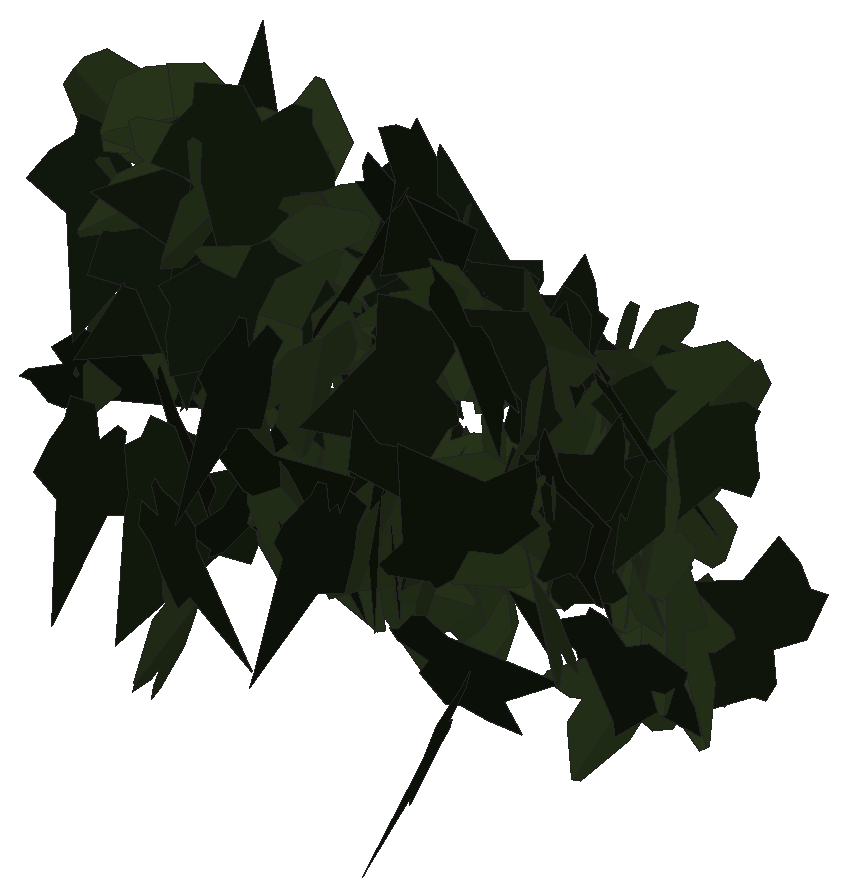
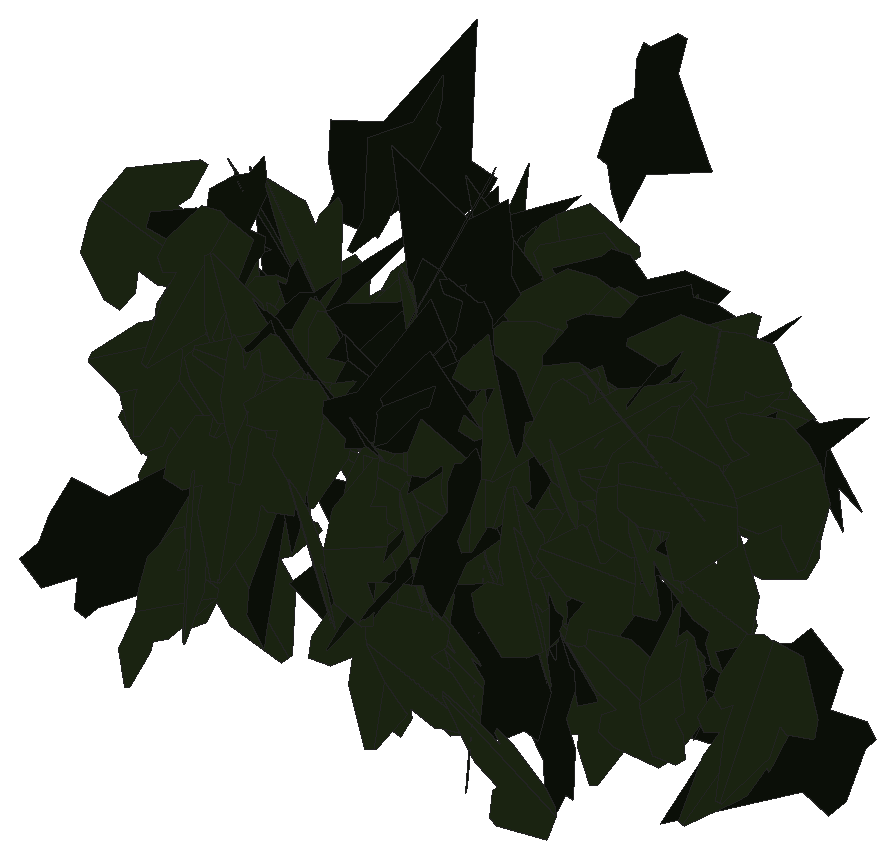
# SketchUp Ruby script. Lengths in inches.
U = 1.inch
M = Sketchup.active_model
def pt(a) = Geom::Point3d.new(a.map { |v| v * U })
def face(e, loops, mat)
  f = e.add_face(loops[0].map { |a| pt(a) })
  loops[1..].each { |l| e.add_face(l.map { |a| pt(a) }).erase! }
  f.material = f.back_material = mat if mat
  f
end
# faces: each face lists its corners as indices into pts; further lists are holes
def faces(e, pts, list, mat = nil) = list.each { |f| face(e, (f[0].is_a?(Array) ? f : [f]).map { |l| l.map { |i| pts[i] } }, mat) }
# xy, xz, yz: faces in a plane at the given z, y or x. An outline is a flat list of corners, or four numbers for a rectangle; further outlines are holes
def ring(l) = l.size == 4 ? [[l[0], l[1]], [l[2], l[1]], [l[2], l[3]], [l[0], l[3]]] : l.each_slice(2).to_a
def flat(e, list, mat, &to3) = list.each { |f| face(e, (f[0].is_a?(Array) ? f : [f]).map { |l| ring(l).map { |u, v| to3.(u, v) } }, mat) }
def xy(e, z, list, mat = nil) = flat(e, list, mat) { |x, y| [x, y, z] }
def xz(e, y, list, mat = nil) = flat(e, list, mat) { |x, z| [x, y, z] }
def yz(e, x, list, mat = nil) = flat(e, list, mat) { |y, z| [x, y, z] }
def lines(e, pts, list) = list.each { |a, b| e.add_line(pt(pts[a]), pt(pts[b])) }
# prism: a flat outline (further loops are holes) pulled along v
def prism(e, loops, v, mat = nil)
  f = face(e, loops, mat); d = Geom::Vector3d.new(v.map { |x| x * U })
  f.pushpull(f.normal.samedirection?(d) ? d.length : -d.length)
end
def box(e, o, s, mat = nil) = prism(e, [[o, [o[0] + s[0], o[1], o[2]], [o[0] + s[0], o[1] + s[1], o[2]], [o[0], o[1] + s[1], o[2]]]], [0, 0, s[2]], mat)
def at(x, y, z, deg = 0) = Geom::Transformation.translation(pt([x, y, z])) * Geom::Transformation.rotation(ORIGIN, Z_AXIS, deg.degrees)
def axes(o, x, y, z) = Geom::Transformation.new([*x, 0, *y, 0, *z, 0, *pt(o).to_a, 1])
def part(name) = M.definitions.add(name)
# library, detail: a bought-in or finely detailed component or shape, given as its bounding box
def library(name, o, s) = part(name).tap { |d| box(d.entities, o, s) }
def detail(e, o, s) = box(e.add_group.entities, o, s)
def put(e, d, t, mat = nil) = e.add_instance(d, t).tap { |i| i.material = mat if mat }
def group(e, t, mat = nil) = e.add_group.tap { |g| g.transformation = t; g.material = mat if mat }.entities
root = M.entities
M.materials.add("efeu1").color = [18, 25, 13]
M.materials.add("efeu2").color = [43, 57, 29]
c1 = part("ivyleaf_9")
p = [[1.54,2.16,1.25],[1.36,2.04,1.19],[-0.21,0.99,0.68],[-0.71,1.11,0.82],[-0.85,0.86,0.67],[-0.8,0.17,0.21],
  [-0.9,-0.01,0.1],[-0.67,-0.16,-0.02],[-0.08,-0.08,-0.05],[-0.03,-0.6,-0.4],[0.65,-0.88,-0.66],[0.83,-0.6,-0.49],
  [1.29,-0.42,-0.43],[1.8125,-0.07,-0.26],[1.21,0.44,0.15]]
faces(c1.entities,p,[[0,1,2,3,4,5,6,7,8,9,10,11,12,13,14]],"efeu1")
c2 = part("ivyleaf_10")
p = [[0,0.5,-0.03],[-0.0625,2.02,-0.43],[-0.19,2.01,-0.46],[-0.54,1.05,-0.29],[-0.52,0.625,-0.18],[-0.83,0.76,-0.28],
  [-1.16,0.64,-0.33],[-1.15,0.33,-0.24],[-0.77,-0.39,0.02],[-0.3,-0.51,0.16],[0.04,-0.48,0.23],[-0.02,2.01,-0.4375],
  [-0.06,2.01,-0.43],[0.04,-0.49,0.23],[0.67,-0.49,0.14],[1.38,0.36,-0.2],[1.375,0.51,-0.24],[0.81,0.65,-0.19],
  [0.62,0.59,-0.15],[0.6,1.09,-0.28],[0.5,1.23,-0.31]]
faces(c2.entities,p,[[0,1,2,3,4,5,6,7,8,9,10],[11,12,0,13,14,15,16,17,18,19,20]],"efeu2")
put(root,c1,axes([24.57,221.07,202.14],[-0.09691,0.11705,-0.47635],[0.32444,-0.34888,-0.15173],[-0.3679,-0.3385,-0.00833]))
put(root,c1,axes([26.43,221.56,200.85],[0.23064,0.14659,0.41871],[-0.35682,-0.21911,0.27326],[0.2636,-0.42485,0.00354]))
put(root,c1,axes([26.27,221.46,199.16],[-0.33973,0.2703,-0.24804],[0.19417,-0.15434,-0.43414],[-0.31126,-0.3913,-0.0001]))
put(root,c1,axes([22.63,221.6,200.39],[-0.392,0.00104,-0.31037],[0.31035,-0.00523,-0.39199],[-0.00406,-0.49997,0.00346]))
put(root,c1,axes([23.41,221.48,200.03],[0.38075,-0.26764,-0.18274],[-0.1457,0.11048,-0.46537],[0.28948,0.40763,0.00614]))
put(root,c1,axes([24.56,222.1,200.1875],[-0.09012,0.12809,-0.47484],[0.30184,-0.36673,-0.15621],[-0.38829,-0.3148,-0.01123]))
put(root,c2,axes([22.77,222.49,198.5],[0.02406,-0.01061,0.49931],[0.25277,-0.43088,-0.02133],[0.43073,0.25344,-0.01538]))
put(root,c1,axes([24.92,222.48,200.85],[0.32631,-0.26668,-0.26908],[0.21233,-0.16537,0.42139],[-0.31375,-0.38927,0.00533]))
put(root,c2,axes([24.31,222.28,201.49],[-0.06314,-0.49578,-0.01462],[0.00371,0.01426,-0.49978],[0.49598,-0.06322,0.00188]))
put(root,c2,axes([23.6,222.47,200.13],[-0.00544,-0.03351,0.49885],[0.48903,-0.10413,-0.00166],[0.10401,0.48789,0.0339]))
put(root,c1,axes([23.73,222.49,199.88],[-0.04913,-0.10947,0.48539],[0.37833,-0.32503,-0.03501],[0.3232,0.36383,0.11477]))
put(root,c2,axes([26.6,222.29,200.14],[-0.39479,0.26822,0.14899],[-0.12851,0.07592,-0.4772],[-0.27861,-0.41508,0.00899]))
put(root,c1,axes([24.99,222.89,201.24],[-0.12512,-0.20006,0.44082],[-0.23562,-0.37257,-0.23596],[0.42288,-0.26678,-0.00105]))
put(root,c2,axes([26.0625,222.65,200.23],[-0.29048,-0.01059,-0.40683],[-0.40343,-0.05821,0.28957],[-0.05349,0.49649,0.02528]))
put(root,c1,axes([25.44,222.84,201.9],[0.14414,-0.36963,0.30429],[0.1142,-0.28207,-0.39673],[0.46495,0.18387,0.00311]))
put(root,c1,axes([23.3125,222.56,201.67],[-0.09559,-0.28994,-0.39598],[0.20677,0.34207,-0.30038],[0.44509,-0.22118,0.05451]))
put(root,c1,axes([26.33,222.91,200.39],[0.01152,-0.04501,0.49784],[0.22807,-0.44264,-0.0453],[0.4448,0.22813,0.01034]))
put(root,c1,axes([26.9375,222.47,200.83],[-0.15217,0.3003,0.36968],[-0.20182,0.31087,-0.3356],[-0.43141,-0.25135,0.0266]))
put(root,c2,axes([23.8,222.53,201.51],[0.01823,0.25613,0.42903],[-0.0222,0.42931,-0.25535],[-0.49917,-0.00974,0.02703]))
put(root,c1,axes([25.01,222.92,198.69],[0.37136,0.12869,-0.30908],[0.29069,0.10508,0.39301],[0.16611,-0.47159,0.00323]))
put(root,c2,axes([25.51,223.11,200.35],[-0.25756,-0.30037,0.30568],[-0.19149,-0.2384,-0.3956],[0.3834,-0.32085,0.00777]))
put(root,c2,axes([25.02,223.08,199.82],[0.17128,-0.46277,0.08069],[0.0265,-0.07623,-0.49344],[0.469,0.17331,-0.00159]))
put(root,c2,axes([23.33,223.08,201.46],[-0.36114,-0.20204,0.28064],[-0.24118,-0.14364,-0.41377],[0.24781,-0.43422,0.00629]))
put(root,c1,axes([26.11,223,200.01],[-0.18723,0.09637,0.45349],[0.38828,-0.23465,0.21018],[0.25334,0.43087,0.01303]))
put(root,c2,axes([22.27,223.52,201.58],[-0.04686,0.03245,0.49674],[0.23524,-0.43827,0.05082],[0.43871,0.23847,0.0258]))
put(root,c2,axes([26.26,222.9,200.375],[0.02665,-0.09856,-0.48946],[-0.11961,0.47463,-0.10209],[0.48475,0.12253,0.00172]))
put(root,c2,axes([25.86,222.98,200.0625],[0.02246,-0.03118,0.49852],[0.31264,0.39007,0.01031],[-0.38955,0.31125,0.03702]))
put(root,c1,axes([26.74,223.18,199.29],[0.27378,0.17613,-0.3795],[-0.3334,-0.18215,-0.32506],[-0.25276,0.43104,0.0177]))
put(root,c1,axes([22.83,223.34,199.03],[0.23501,0.34912,0.26997],[-0.15043,-0.22418,0.42085],[0.4149,-0.27903,-0.00034]))
put(root,c1,axes([22.1,223.56,199.04],[-0.31146,-0.39073,0.01794],[-0.01027,-0.01475,-0.49968],[0.39101,-0.31163,0.00116]))
put(root,c2,axes([27.02,223.21,200.2],[0.4115,-0.25934,0.1158],[-0.09543,0.06576,0.48638],[-0.26751,-0.42239,0.00462]))
put(root,c1,axes([23.73,223.29,201.27],[0.05953,0.43676,0.23599],[-0.03068,-0.23399,0.4408],[0.49549,-0.06696,-0.00106]))
put(root,c2,axes([24.43,223.35,201.19],[-0.11502,-0.48636,-0.01509],[0.00462,0.01441,-0.49977],[0.48657,-0.11511,0.00118]))
put(root,c2,axes([22.01,223.63,201.76],[-0.10832,-0.1658,0.45911],[-0.21727,-0.40475,-0.19743],[0.43711,-0.24227,0.01564]))
put(root,c2,axes([23.21,223.5,199.93],[0.3796,-0.2206,0.23925],[0.20879,-0.11687,-0.43903],[0.24963,0.43322,0.00339]))
put(root,c1,axes([21.89,223.62,199.23],[0.06409,-0.13447,0.47729],[0.18379,-0.44054,-0.1488],[0.46056,0.19452,-0.00704]))
put(root,c1,axes([21.89,223.77,200.7],[0.11036,-0.23639,-0.42655],[0.16608,-0.39297,0.26075],[-0.45852,-0.19923,-0.00822]))
put(root,c2,axes([23.9,223.43,200.14],[-0.29406,-0.40134,0.04954],[-0.02501,-0.04309,-0.49751],[0.40361,-0.29507,0.00527]))
put(root,c2,axes([23.97,223.44,198.95],[-0.14176,-0.47431,0.07024],[0.03744,0.06207,0.49472],[-0.47802,0.14552,0.01792]))
put(root,c2,axes([26.83,223.51,199.77],[0.45599,-0.10981,0.17326],[0.16951,-0.03611,-0.469],[0.11551,0.48645,0.0043]))
put(root,c2,axes([23.3,223.25,201.71],[-0.27791,-0.24485,-0.33588],[0.26526,0.20659,-0.37008],[0.32,-0.38389,0.01507]))
put(root,c2,axes([26.5,223.6,198.74],[-0.25217,-0.36102,0.2368],[-0.1187,-0.20569,-0.44],[0.41512,-0.27813,0.01803]))
put(root,c1,axes([21.2,223.8,201.39],[-0.14292,-0.4697,0.09465],[-0.02994,-0.08982,-0.49095],[0.4782,-0.146,-0.00245]))
put(root,c1,axes([26.4375,223.43,201.39],[0.44346,-0.21792,-0.07648],[-0.0644,0.04232,-0.49403],[0.22179,0.44802,0.00947]))
put(root,c1,axes([22.26,223.86,201.35],[0.03113,-0.44016,-0.23513],[0.03702,-0.23291,0.44089],[-0.49766,-0.04486,0.01809]))
put(root,c2,axes([26.28,223.67,199.82],[0.06239,-0.03223,0.49504],[0.46972,-0.15668,-0.0694],[0.1596,0.47372,0.01072]))
put(root,c1,axes([23.77,223.6875,199.84],[-0.16911,0.04101,-0.46874],[0.46015,-0.08967,-0.17385],[-0.09832,-0.49018,-0.00741]))
put(root,c2,axes([23.31,223.8,199.83],[-0.11938,-0.32406,0.36157],[-0.09517,-0.34949,-0.34467],[0.47612,-0.15112,0.02176]))
put(root,c1,axes([21.8,223.69,201.2],[-0.04827,-0.48838,-0.09568],[0.00727,0.09543,-0.49076],[0.49761,-0.04877,-0.00211]))
put(root,c2,axes([25.73,223.62,200.51],[-0.07266,-0.00345,-0.49468],[0.45896,-0.18704,-0.06611],[-0.18459,-0.46368,0.03035]))
put(root,c1,axes([27.0625,223.77,201.32],[-0.40803,-0.28646,-0.03803],[0.03097,0.02208,-0.49855],[0.28731,-0.40921,-0.00028]))
put(root,c2,axes([25.54,223.68,201.38],[-0.21162,0.04064,0.45118],[0.43692,-0.11321,0.21513],[0.11964,0.48532,0.0124]))
put(root,c2,axes([24.9375,223.9,199.87],[-0.03448,0.02916,0.49796],[0.22495,-0.44459,0.04161],[0.4452,0.2269,0.01754]))
put(root,c2,axes([25.66,223.3125,200.84],[0.0502,-0.28491,-0.4078],[0.00392,0.41009,-0.28603],[0.49746,0.02552,0.04341]))
put(root,c2,axes([24.69,223.6,201.46],[0.22115,-0.00602,-0.44839],[-0.44464,0.0619,-0.22014],[0.05816,0.49612,0.02203]))
put(root,c2,axes([26.8,223.625,199.36],[0.422,0.0416,0.26493],[0.26284,0.03387,-0.42399],[-0.05322,0.49711,0.00672]))
put(root,c1,axes([23.62,223.79,200.375],[-0.01684,0.01064,0.4996],[0.28707,-0.40896,0.01839],[0.40903,0.28746,0.00766]))
put(root,c1,axes([24.12,224.03,202.125],[-0.03368,-0.27691,0.41495],[-0.01104,-0.41538,-0.2781],[0.49874,-0.0279,0.02187]))
put(root,c1,axes([24.02,223.85,201.8],[-0.0348,-0.13889,0.47906],[0.34212,-0.3561,-0.0784],[0.36297,0.32233,0.11982]))
put(root,c1,axes([22.47,223.875,202.23],[-0.20199,-0.44696,-0.09707],[0.03957,0.08864,-0.49049],[0.45567,-0.20583,-0.00043]))
put(root,c1,axes([25.67,223.99,201.01],[-0.03747,-0.48223,-0.12669],[-0.01032,-0.12627,0.48368],[-0.49849,0.03886,-0.00049]))
put(root,c2,axes([27.12,224,201.51],[-0.10257,-0.32492,0.36593],[-0.08665,-0.35592,-0.34032],[0.48163,-0.13322,0.01671]))
put(root,c2,axes([21.81,223.87,201.75],[-0.30306,-0.28903,0.27317],[-0.17092,-0.21544,-0.41758],[0.35909,-0.34648,0.03178]))
put(root,c1,axes([24.84,223.9,199.28],[0.29099,-0.36775,0.17345],[0.10841,-0.13539,-0.46895],[0.39188,0.31053,0.00094]))
put(root,c2,axes([23.93,223.88,198.625],[0.07115,-0.10717,-0.48317],[0.42113,-0.2433,0.11598],[-0.25997,-0.42346,0.05564]))
put(root,c1,axes([22.16,224.15,201.66],[-0.09899,-0.38792,0.29953],[-0.081,-0.28843,-0.40031],[0.48336,-0.12778,-0.00574]))
put(root,c2,axes([24.3125,223.67,199.76],[0.23165,-0.01769,-0.44275],[0.44163,0.04992,0.22906],[0.0361,-0.49719,0.03876]))
put(root,c2,axes([22.76,223.8125,198.88],[-0.1652,0.00002,-0.47192],[0.45542,-0.13106,-0.15943],[-0.12371,-0.48252,0.04328]))
put(root,c2,axes([20.99,223.6875,200.9],[-0.08265,-0.05095,0.49048],[0.45344,0.1876,0.0959],[-0.19381,0.46066,0.0152]))
put(root,c2,axes([24.85,223.99,200.89],[-0.29107,-0.3097,-0.26337],[-0.18139,-0.19095,0.42501],[-0.36383,0.34296,-0.00119]))
put(root,c2,axes([26,223.61,200.94],[-0.10952,-0.38885,-0.29462],[0.1382,0.26486,-0.40094],[0.46788,-0.16925,0.04946]))
put(root,c1,axes([24.35,224.2,199.53],[-0.08273,-0.35518,0.34206],[-0.0376,-0.34128,-0.36347],[0.49167,-0.08586,0.02976]))
put(root,c2,axes([24.4375,223.9,199.82],[0.23035,-0.44235,0.0356],[0.02091,-0.02925,-0.49871],[0.44329,0.23124,0.00503]))
put(root,c2,axes([23.4,223.71,201.15],[-0.27991,-0.36859,-0.18918],[0.11606,0.1494,-0.46283],[0.39772,-0.30302,0.00192]))
put(root,c2,axes([21.61,223.8,202.24],[0.43397,0.22226,0.11075],[0.09467,0.05808,-0.48751],[-0.22958,0.4441,0.00833]))
put(root,c2,axes([22.47,223.7,200.125],[-0.30144,0.32664,-0.22901],[-0.15328,0.17016,0.44447],[0.3683,0.33816,-0.00245]))
put(root,c1,axes([25.54,224,200.21],[-0.04433,-0.00128,-0.49803],[0.49711,-0.03047,-0.04417],[-0.03023,-0.49907,0.00397]))
put(root,c2,axes([21.33,223.94,200.09],[-0.03486,-0.03651,0.49744],[0.49781,-0.03371,0.03241],[0.03117,0.49752,0.03871]))
put(root,c2,axes([24.31,223.85,201.11],[0.26658,-0.41742,0.06855],[-0.03728,0.05752,0.49528],[-0.42136,-0.26917,-0.00046]))
put(root,c2,axes([26.76,223.96,200.32],[-0.3211,-0.09402,0.37156],[-0.34603,-0.13731,-0.33378],[0.1648,-0.47149,0.02312]))
put(root,c2,axes([22.03,224.13,200.92],[0.15564,-0.41687,0.22801],[0.10164,-0.20517,-0.44449],[0.46416,0.18471,0.02087]))
put(root,c2,axes([23.86,223.91,200.92],[-0.23665,-0.43747,-0.05117],[0.02354,0.04544,-0.49737],[0.43982,-0.23781,-0.00091]))
put(root,c1,axes([24.43,223.79,201.34],[0.03153,-0.1783,-0.46607],[0.20194,0.43161,-0.15145],[0.45632,-0.17868,0.09922]))
put(root,c2,axes([24.65,223.91,198.93],[-0.41319,-0.27836,-0.04232],[0.03508,0.02367,-0.49821],[0.27936,-0.41468,-0.00003]))
put(root,c1,axes([25.51,223.74,200.8125],[-0.05749,0.07885,0.49039],[-0.26605,0.41198,-0.09743],[-0.41942,-0.27214,-0.00541]))
put(root,c1,axes([23.5625,223.91,201.39],[-0.00481,-0.33949,-0.36705],[0.09064,0.36039,-0.33452],[0.49169,-0.06976,0.05808]))
put(root,c1,axes([23.74,224.33,200.33],[0.00408,-0.05075,-0.4974],[0.32087,-0.3812,0.04153],[-0.38344,-0.31954,0.02946]))
put(root,c1,axes([23.12,224.12,199.24],[0.25496,0.00727,-0.43005],[0.42579,0.06638,0.25356],[0.06078,-0.49552,0.02766]))
put(root,c2,axes([23.03,223.86,200.82],[-0.07996,0.05596,-0.49038],[-0.38944,0.29804,0.09751],[0.30322,0.39755,-0.00408]))
put(root,c2,axes([24.68,224.41,199.72],[0.08751,-0.17447,0.46033],[0.17323,-0.42672,-0.19467],[0.46079,0.19356,-0.01424]))
put(root,c2,axes([23.16,223.97,201.68],[-0.41701,-0.2231,-0.16226],[0.14518,0.0726,-0.47292],[0.23458,-0.44154,0.00423]))
put(root,c2,axes([24.58,224.01,198.6875],[0.17774,-0.03605,-0.46595],[-0.44569,0.1369,-0.18061],[0.1406,0.47954,0.01653]))
put(root,c1,axes([22.72,224.26,198.9],[0.09451,-0.05304,-0.48811],[0.48899,-0.03459,0.09844],[-0.04421,-0.49597,0.04533]))
put(root,c1,axes([23.86,223.84,199.28],[0.11979,-0.02438,-0.48483],[-0.45604,0.16548,-0.121],[0.16636,0.47119,0.01741]))
put(root,c1,axes([23.47,224.1875,201.72],[-0.06096,-0.07882,-0.48997],[0.48274,0.10508,-0.07696],[0.11511,-0.48244,0.06329]))
put(root,c2,axes([22.39,223.82,200.84],[-0.16939,-0.23436,-0.4079],[0.23975,0.33001,-0.28916],[0.40475,-0.29355,0.00057]))
put(root,c2,axes([23.32,224.07,200.03],[0.33809,-0.32832,-0.16704],[-0.10887,0.12755,-0.47104],[0.35192,0.35488,0.01476]))
put(root,c1,axes([20.63,223.79,199.48],[0.39899,0.23091,0.19363],[0.16025,0.1095,-0.46079],[-0.2552,0.42976,0.01337]))
put(root,c2,axes([26.05,224.04,199.91],[-0.4984,0.02986,0.02665],[-0.02685,-0.00245,-0.49927],[-0.02969,-0.4991,0.00404]))
put(root,c2,axes([23.08,224.2,199.61],[0.03016,-0.49395,-0.07141],[0.02065,-0.07025,0.49461],[-0.49866,-0.03279,0.01616]))
put(root,c2,axes([21.95,224.48,201.24],[-0.07187,-0.10494,0.48355],[0.06746,-0.48614,-0.09547],[0.49019,0.05152,0.08404]))
put(root,c2,axes([26.34,223.9,201.48],[-0.11071,-0.31564,-0.37163],[0.11267,0.35422,-0.33442],[0.47439,-0.15779,-0.0073]))
put(root,c2,axes([25.74,224.26,200.69],[-0.4266,-0.07688,0.2492],[0.25471,-0.02027,0.42978],[-0.05598,0.49364,0.05646]))
put(root,c2,axes([22.44,223.94,200.04],[0.09001,-0.30902,0.38263],[-0.05047,0.38112,0.31968],[-0.48924,-0.09617,0.03742]))
put(root,c1,axes([24,224.32,201.56],[0.34628,-0.30022,0.1999],[0.15059,-0.13146,-0.4583],[0.32774,0.37761,-0.00063]))
put(root,c2,axes([20.5625,224.24,201.75],[-0.30555,0.08287,-0.387],[0.37057,-0.11178,-0.31652],[-0.13898,-0.48025,0.00689]))
put(root,c2,axes([25.17,224.09,200.77],[-0.08667,-0.05894,0.48889],[0.41712,0.25504,0.1047],[-0.26172,0.426,0.00496]))
put(root,c2,axes([25.17,224.32,199.88],[0.35256,-0.35452,0.00417],[0.00297,-0.00292,-0.49998],[0.35453,0.35258,0.00004]))
put(root,c2,axes([22.51,224.5,201.49],[0.19164,-0.37663,0.26725],[0.14134,-0.22763,-0.42214],[0.43966,0.23735,0.01922]))
put(root,c1,axes([24.13,224.14,200.6875],[-0.48097,-0.03234,0.13274],[0.13251,0.00778,0.48206],[-0.03324,0.49889,0.00108]))
put(root,c1,axes([27.04,224.61,198.81],[0.0019,0.04011,0.49839],[-0.40432,-0.29308,0.02513],[0.29415,-0.40311,0.03132]))
put(root,c1,axes([24.28,224.28,200.9],[-0.35514,-0.28506,0.20645],[0.18885,0.09316,0.45349],[-0.29701,0.40008,0.0415]))
put(root,c2,axes([21.74,224.3,199.27],[-0.25348,-0.07678,0.42409],[0.40089,0.13862,0.26471],[-0.15822,0.47423,-0.00871]))
put(root,c2,axes([26.38,224.67,198.77],[0.03662,0.20461,-0.45475],[-0.05522,-0.4515,-0.20759],[-0.49559,0.06543,-0.01047]))
put(root,c1,axes([25.33,224.15,200.95],[-0.18085,0.26056,0.38653],[-0.25388,0.29266,-0.31607],[-0.39095,-0.31058,0.02645]))
put(root,c2,axes([21.44,224.73,199.73],[0.04635,-0.07554,0.49208],[0.25553,-0.42054,-0.08862],[0.42727,0.2597,-0.00038]))
put(root,c2,axes([24.94,224.33,200.85],[0.34611,0.35167,0.08085],[0.05613,0.05819,-0.49342],[-0.35645,0.35063,0.0008]))
put(root,c2,axes([26.27,224.2,199.42],[0.12596,-0.35859,-0.32488],[-0.06537,0.32002,-0.37857],[0.47944,0.13784,0.03374]))
put(root,c1,axes([22.07,224.13,201.43],[-0.42975,0.22939,-0.11266],[-0.10071,0.05056,0.48714],[0.23488,0.44139,0.00275]))
put(root,c2,axes([22.88,224.49,198.3],[0.19668,-0.16865,-0.42764],[0.40667,-0.15304,0.24739],[-0.21434,-0.44512,0.07697]))
put(root,c2,axes([22.3125,224.65,201.5],[0.12245,0.23019,0.42663],[-0.19019,-0.38194,0.26067],[0.44591,-0.22612,-0.00597]))
put(root,c2,axes([20.81,224.23,199.9375],[-0.08342,-0.37713,-0.31751],[0.047,0.31447,-0.38587],[0.49075,-0.09423,-0.01702]))
put(root,c2,axes([20.85,224.21,199.58],[-0.14148,-0.30558,-0.36961],[0.16899,0.32887,-0.33658],[0.44881,-0.22015,0.01022]))
put(root,c2,axes([21.28,224.41,201.32],[-0.0295,-0.03431,-0.49795],[0.49889,-0.01734,-0.02836],[-0.01532,-0.49852,0.03525]))
put(root,c2,axes([26.61,224.11,200.68],[0.03629,0.13495,-0.48007],[0.0996,0.46969,0.13956],[0.48863,-0.10576,0.00721]))
put(root,c2,axes([25.39,224.86,200.74],[0.015,-0.05527,-0.49671],[0.07298,-0.49136,0.05688],[-0.49442,-0.07421,-0.00668]))
